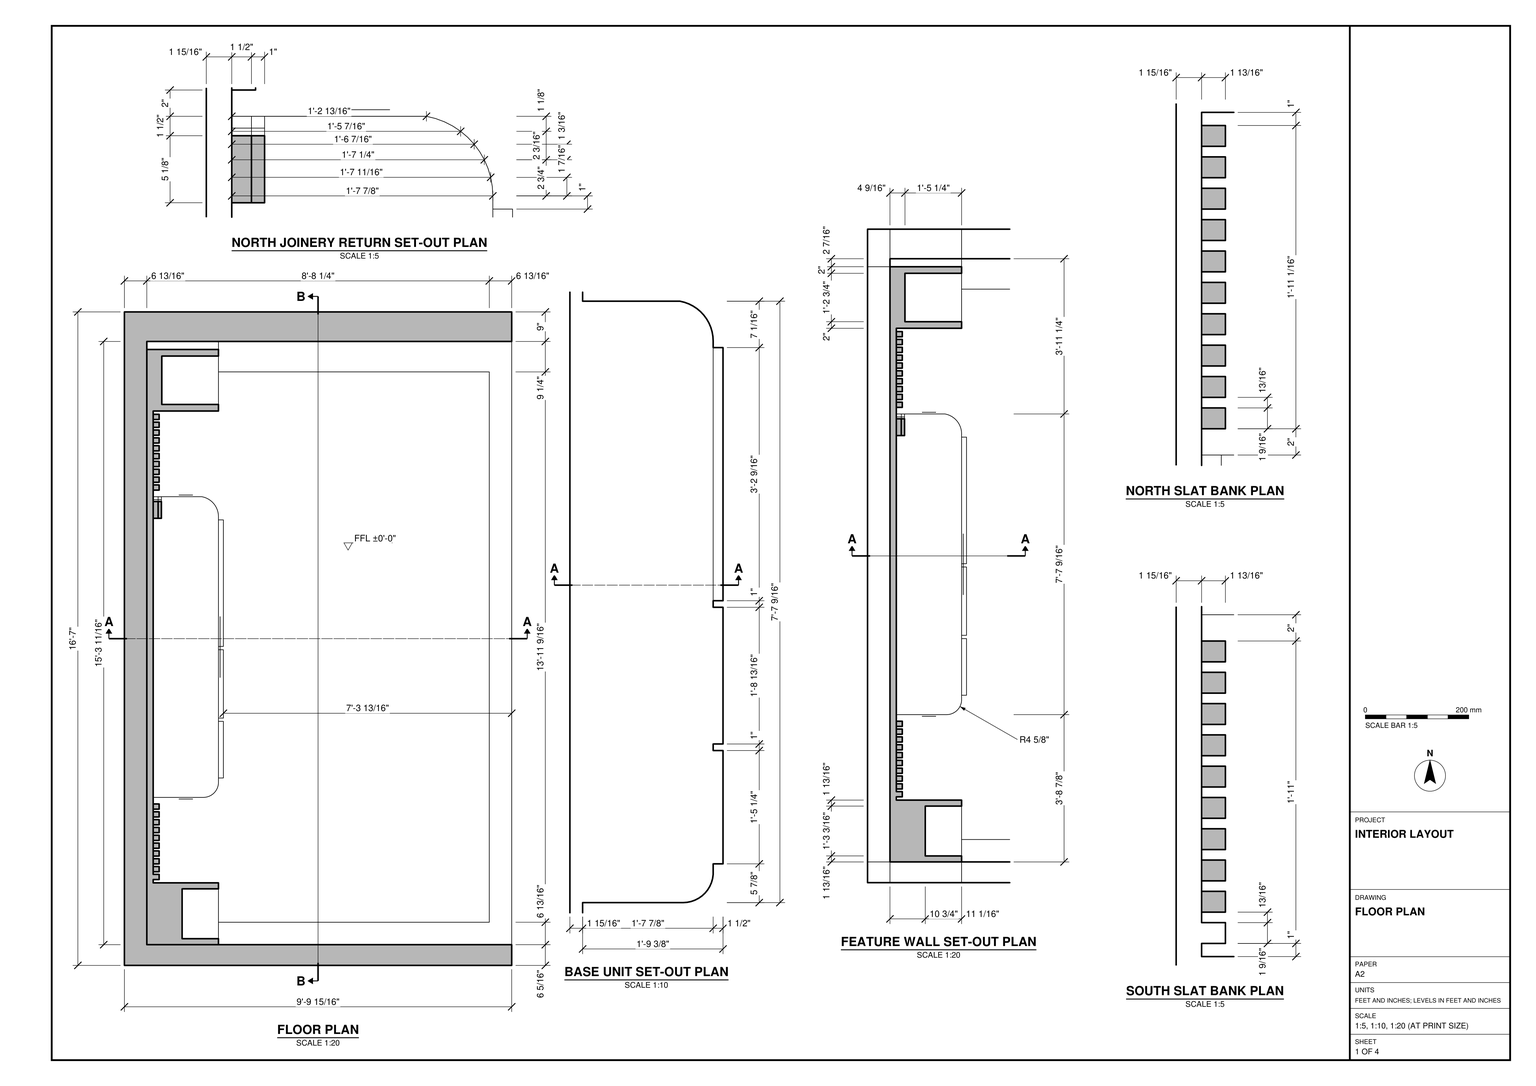
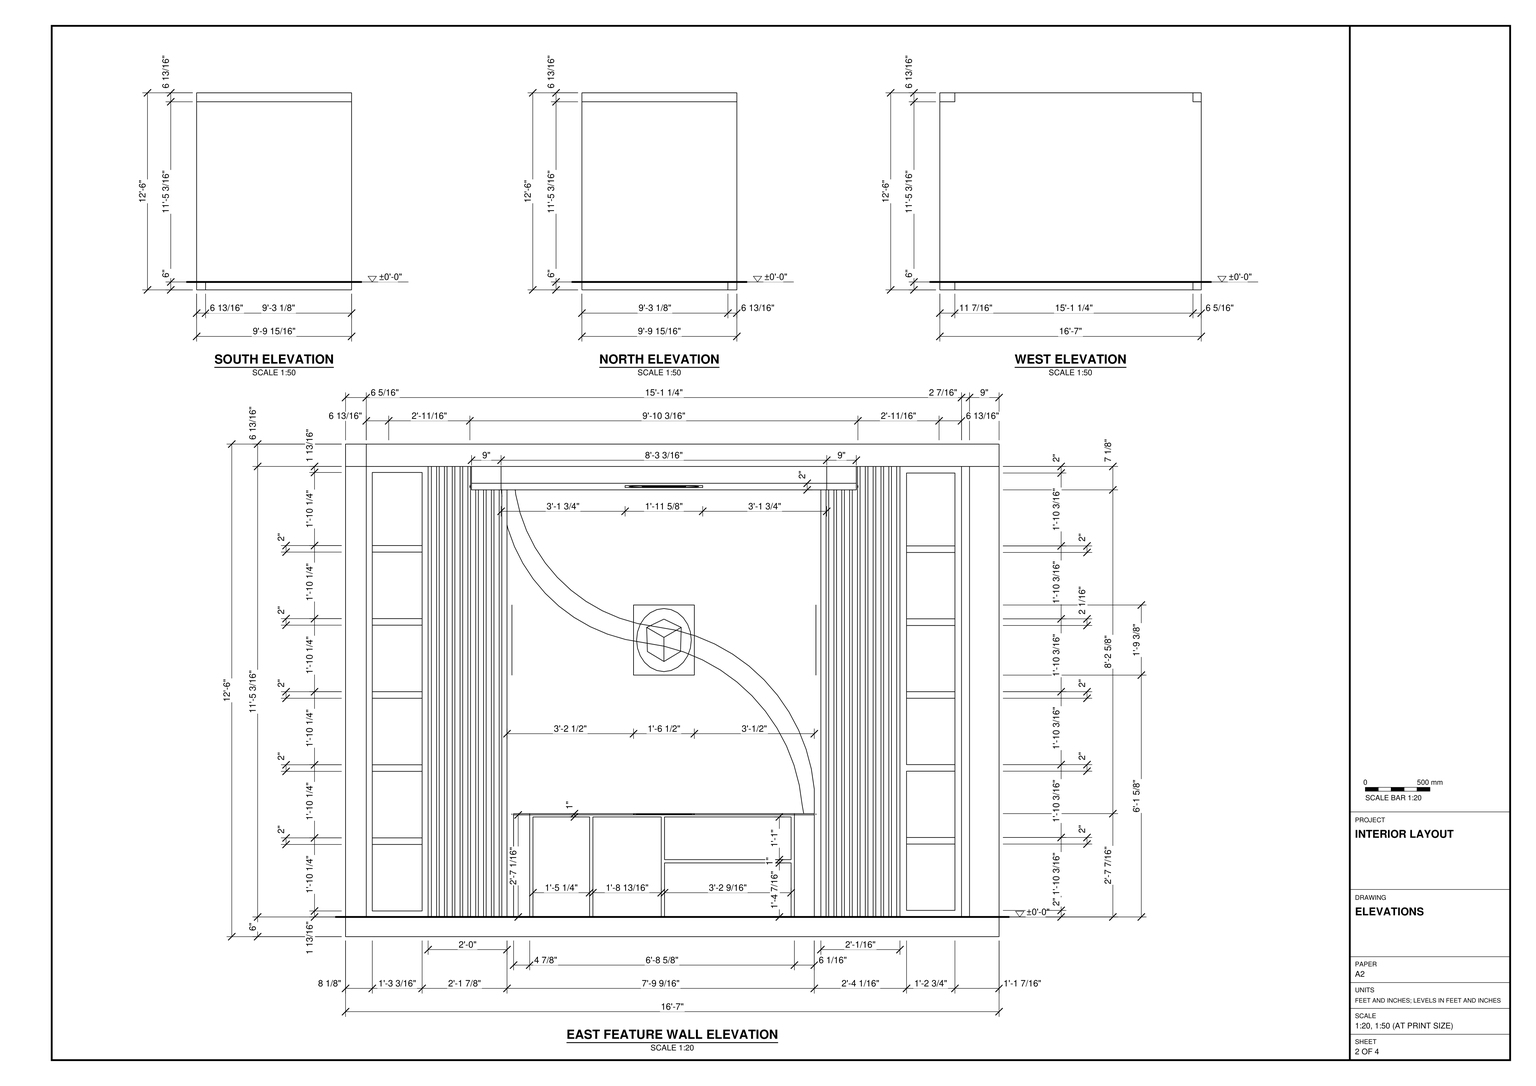
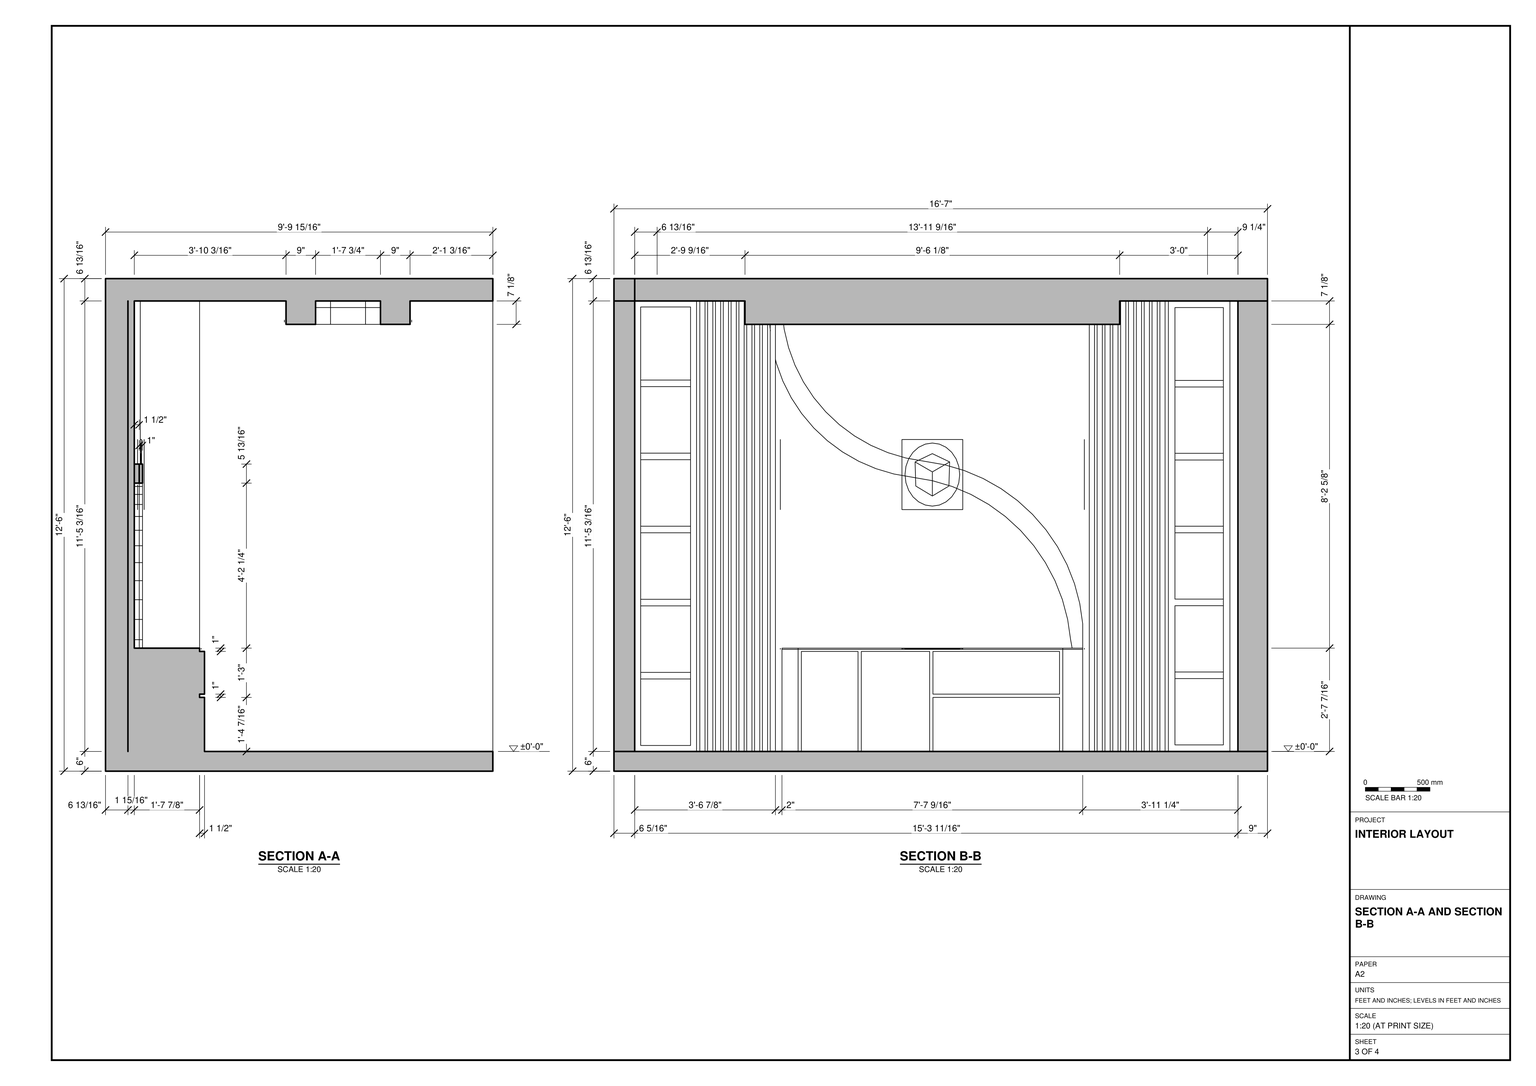
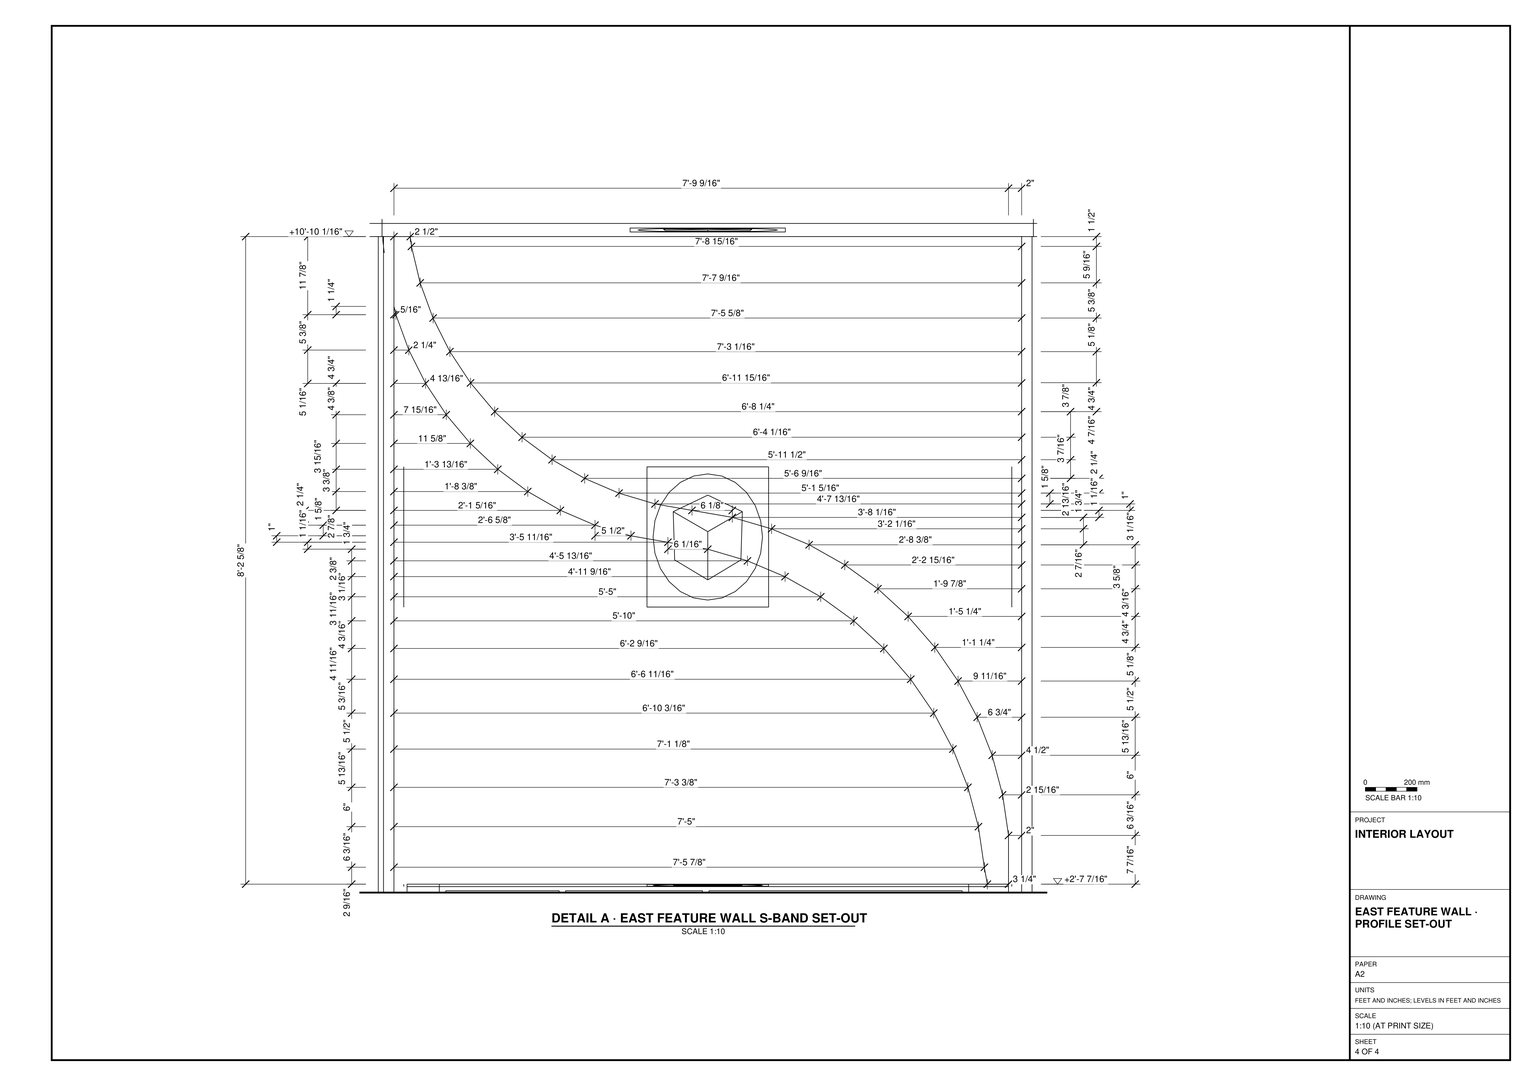
Build the room and its fitted joinery in SketchUp from task_files/diagram_01.pdf. Work in feet and inches. Set the finished floor at ±0'-0". The room shell measures 9'-9 15/16" east to west, 16'-7" north to south and 12'-6" high overall, including the floor and ceiling slabs.

Model the long west wall and the north and south end walls at their drawn thicknesses, leaving the east side open as shown in plan. Use the two sections to set the slab thicknesses and the position, depth and length of the ceiling projections. Keep the floor area in front of the joinery clear.

Build the east-facing feature wall using the elevation for the shelf heights and cabinet divisions, and the enlarged plans for the profiles. At each end, form a tall bank of open shelves with its own return depth. Place the closely spaced vertical slats between the shelves and the central panel. Run the curved band across the panel from the upper left to the lower right as seen in elevation, with the small wall-mounted feature near its centre. Below it, model the low base cabinet with its rounded front corners in plan and its divided front as drawn. Decor and loose items may be represented by any suitable library component.

Keep the walls, slabs and each joinery or furniture piece in separate groups or components, and use components for repeated parts such as matching slats. Save one SketchUp model as output_files/feature_wall_with_flanking_shelves_and_base_cabinetry.skp.

# SketchUp Ruby script. Lengths in inches.
U = 1.inch
M = Sketchup.active_model
def pt(a) = Geom::Point3d.new(a.map { |v| v * U })
def face(e, loops, mat)
  f = e.add_face(loops[0].map { |a| pt(a) })
  loops[1..].each { |l| e.add_face(l.map { |a| pt(a) }).erase! }
  f.material = f.back_material = mat if mat
  f
end
# faces: each face lists its corners as indices into pts; further lists are holes
def faces(e, pts, list, mat = nil) = list.each { |f| face(e, (f[0].is_a?(Array) ? f : [f]).map { |l| l.map { |i| pts[i] } }, mat) }
# xy, xz, yz: faces in a plane at the given z, y or x. An outline is a flat list of corners, or four numbers for a rectangle; further outlines are holes
def ring(l) = l.size == 4 ? [[l[0], l[1]], [l[2], l[1]], [l[2], l[3]], [l[0], l[3]]] : l.each_slice(2).to_a
def flat(e, list, mat, &to3) = list.each { |f| face(e, (f[0].is_a?(Array) ? f : [f]).map { |l| ring(l).map { |u, v| to3.(u, v) } }, mat) }
def xy(e, z, list, mat = nil) = flat(e, list, mat) { |x, y| [x, y, z] }
def xz(e, y, list, mat = nil) = flat(e, list, mat) { |x, z| [x, y, z] }
def yz(e, x, list, mat = nil) = flat(e, list, mat) { |y, z| [x, y, z] }
def lines(e, pts, list) = list.each { |a, b| e.add_line(pt(pts[a]), pt(pts[b])) }
# prism: a flat outline (further loops are holes) pulled along v
def prism(e, loops, v, mat = nil)
  f = face(e, loops, mat); d = Geom::Vector3d.new(v.map { |x| x * U })
  f.pushpull(f.normal.samedirection?(d) ? d.length : -d.length)
end
def box(e, o, s, mat = nil) = prism(e, [[o, [o[0] + s[0], o[1], o[2]], [o[0] + s[0], o[1] + s[1], o[2]], [o[0], o[1] + s[1], o[2]]]], [0, 0, s[2]], mat)
def at(x, y, z, deg = 0) = Geom::Transformation.translation(pt([x, y, z])) * Geom::Transformation.rotation(ORIGIN, Z_AXIS, deg.degrees)
def axes(o, x, y, z) = Geom::Transformation.new([*x, 0, *y, 0, *z, 0, *pt(o).to_a, 1])
def part(name) = M.definitions.add(name)
# library, detail: a bought-in or finely detailed component or shape, given as its bounding box
def library(name, o, s) = part(name).tap { |d| box(d.entities, o, s) }
def detail(e, o, s) = box(e.add_group.entities, o, s)
def put(e, d, t, mat = nil) = e.add_instance(d, t).tap { |i| i.material = mat if mat }
def group(e, t, mat = nil) = e.add_group.tap { |g| g.transformation = t; g.material = mat if mat }.entities
root = M.entities
M.materials.add("Marble Black 01 150cm").color = [30, 30, 30]
M.materials.add("Tiles Simple J01 100cm").color = [187, 218, 215]
M.materials.add("Wood Maple 33-40 200cm").color = [215, 177, 122]
M.materials.add("[Color D01]").color = [255, 242, 204]
M.materials.add("[Color F01]").color = [229, 255, 204]
M.materials.add("[Color M04]").color = [142, 142, 142]
c1 = library("Spot Light",[-5.1,-5.1,-11.05],[10.2,10.2,11.05])
c2 = library("Spot Light\#1",[-5.1,-5.1,-11.05],[10.2,10.2,11.05])
c3 = library("Group\#2",[0,0,0],[3,94.07,105.72])
c4 = library("Group\#3",[-0.5,-0.5,0],[20.875,92.57,0.375])
c5 = library("Group\#5",[-0.5,-0.5,0],[38.76,118.17,7.125])
c6 = library("Group\#6",[-0.5,-0.5,0],[20.76,100.17,2])
xy(root,0,[[0,0,0,187.5625,6.83,187.5625,6.83,199,117.9375,199,117.9375,0],[0,187.5625,6.83,199]])
xy(root,6,[[0,0,6.83,6.3125],[6.83,0,28.64,6.3125],[8.77,28.52,10.58,30.11],[8.77,30.9,10.58,32.49],[8.77,33.29,10.58,34.87],
  [8.77,35.67,10.58,37.25],[8.77,38.05,10.58,39.64],[8.77,40.43,10.58,42.02],[8.77,42.81,10.58,44.4],[8.77,45.2,10.58,46.78],
  [8.77,47.58,10.58,49.16],[8.77,144.73,10.58,146.32],[8.77,147.12,10.58,148.71],[8.77,149.51,10.58,151.1],[8.77,151.9,10.58,153.49],
  [8.77,154.29,10.58,155.875],[8.77,156.68,10.58,158.26],[8.77,159.07,10.58,160.65],[8.77,161.46,10.58,163.04],[8.77,163.85,10.58,165.43],
  [8.77,166.23,10.58,167.82],[0,187.5625,6.83,199],[6.83,187.5625,28.64,199]])
xy(root,6,[[28.64,0,117.9375,0,117.9375,199,28.64,199,28.64,180.73,111.11,180.73,111.11,13.14,28.64,13.14],[28.64,13.14,111.11,13.14,111.11,180.73,28.64,180.73,28.64,168.82,8.77,168.82,8.77,167.82,10.58,167.82,10.58,166.23,8.77,166.23,8.77,165.43,10.58,165.43,10.58,163.85,8.77,163.85,8.77,163.04,10.58,163.04,10.58,161.46,8.77,161.46,8.77,160.65,10.58,160.65,10.58,159.07,8.77,159.07,8.77,158.26,10.58,158.26,10.58,156.68,8.77,156.68,8.77,155.875,10.58,155.875,10.58,154.29,8.77,154.29,8.77,153.49,10.58,153.49,10.58,151.9,8.77,151.9,8.77,151.1,10.58,151.1,10.58,149.51,8.77,149.51,8.77,148.71,10.58,148.71,10.58,147.12,8.77,147.12,8.77,146.32,10.58,146.32,10.58,144.73,8.77,144.73,8.77,142.73,23.59,142.73,24.28,142.57,24.95,142.32,25.58,141.99,26.18,141.6,26.72,141.14,27.21,140.62,27.64,140.04,27.99,139.43,28.27,138.77,28.48,138.09,28.6,137.38,28.64,136.67,28.64,135.67,30.14,135.67,30.14,97.13,28.64,97.13,28.64,96.13,30.14,96.13,30.14,75.32,28.64,75.32,28.64,74.32,30.14,74.32,30.14,57.07,28.64,57.07,28.64,55.44,28.55,54.82,28.38,54.22,28.13,53.64,27.81,53.11,27.41,52.62,26.95,52.19,26.4375,51.83,25.88,51.54,25.29,51.33,24.68,51.21,24.05,51.16,8.77,51.16,8.77,49.16,10.58,49.16,10.58,47.58,8.77,47.58,8.77,46.78,10.58,46.78,10.58,45.2,8.77,45.2,8.77,44.4,10.58,44.4,10.58,42.81,8.77,42.81,8.77,42.02,10.58,42.02,10.58,40.43,8.77,40.43,8.77,39.64,10.58,39.64,10.58,38.05,8.77,38.05,8.77,37.25,10.58,37.25,10.58,35.67,8.77,35.67,8.77,34.87,10.58,34.87,10.58,33.29,8.77,33.29,8.77,32.49,10.58,32.49,10.58,30.9,8.77,30.9,8.77,30.11,10.58,30.11,10.58,28.52,8.77,28.52,8.77,27.73,10.58,27.73,10.58,26.14,8.77,26.14,8.77,25.14,28.64,25.14]],"Tiles Simple J01 100cm")
xy(root,7.83,[[17.58,8.14,28.64,13.14],[17.58,13.14,28.64,23.32]],"Marble Black 01 150cm")
xy(root,8,[[11.39,170.82,28.64,180.73],[11.39,180.73,28.64,185.5625]],"Marble Black 01 150cm")
xy(root,22.46,[[28.64,97.13,30.14,135.67]],"Wood Maple 33-40 200cm")
xy(root,23.46,[[28.64,97.13,30.14,135.67]])
xy(root,28.08,[[17.58,8.14,28.64,23.32]],"Marble Black 01 150cm")
xy(root,28.2,[[11.39,170.82,28.64,185.5625]],"Marble Black 01 150cm")
xy(root,30.08,[[17.58,8.14,28.64,23.32]],"Marble Black 01 150cm")
xy(root,30.2,[[11.39,170.82,28.64,185.5625]],"Marble Black 01 150cm")
xy(root,36.46,[[28.64,97.13,30.14,135.67]])
xy(root,36.46,[[28.64,57.07,30.14,74.32],[28.64,75.32,30.14,96.13]],"Wood Maple 33-40 200cm")
xy(root,37.46,[[8.77,51.16,24.05,51.16,24.68,51.21,25.29,51.33,25.88,51.54,26.4375,51.83,26.95,52.19,27.41,52.62,27.81,53.11,28.13,53.64,28.38,54.22,28.55,54.82,28.64,55.44,28.64,136.67,28.6,137.38,28.48,138.09,28.27,138.77,27.99,139.43,27.64,140.04,27.21,140.62,26.72,141.14,26.18,141.6,25.58,141.99,24.95,142.32,24.28,142.57,23.59,142.73,8.77,142.73]],"Wood Maple 33-40 200cm")
xy(root,50.34,[[17.58,8.14,28.64,23.32]],"Marble Black 01 150cm")
xy(root,52.34,[[17.58,8.14,28.64,23.32]],"Marble Black 01 150cm")
xy(root,52.4,[[11.39,170.82,28.64,185.5625]],"Marble Black 01 150cm")
xy(root,72.59,[[17.58,8.14,28.64,23.32]],"Marble Black 01 150cm")
xy(root,72.6,[[11.39,170.82,28.64,185.5625]],"Marble Black 01 150cm")
xy(root,74.59,[[17.58,8.14,28.64,23.32],[11.39,170.82,28.64,185.5625]],"Marble Black 01 150cm")
xy(root,94.75,[[11.39,170.82,28.64,185.5625]],"Marble Black 01 150cm")
xy(root,94.85,[[17.58,8.14,28.64,23.32]],"Marble Black 01 150cm")
xy(root,96.79,[[11.39,170.82,28.64,185.5625]],"Marble Black 01 150cm")
xy(root,96.85,[[17.58,8.14,28.64,23.32]],"Marble Black 01 150cm")
xy(root,116.99,[[11.39,170.82,28.64,185.5625]],"Marble Black 01 150cm")
xy(root,117.11,[[17.58,8.14,28.64,23.32]],"Marble Black 01 150cm")
xy(root,118.99,[[11.39,170.82,28.64,185.5625]])
xy(root,119.11,[[17.58,8.14,28.64,23.32]],"Marble Black 01 150cm")
xy(root,141.1875,[[11.39,170.82,28.64,180.73],[11.39,180.73,28.64,185.5625]],"Marble Black 01 150cm")
xy(root,141.36,[[17.58,8.14,28.64,13.14],[17.58,13.14,28.64,23.32]],"Marble Black 01 150cm")
xy(root,143.1875,[[0,0,6.83,6.3125],[6.83,0,28.64,6.3125],[8.77,28.52,10.58,30.11],[8.77,30.9,10.58,32.49],[8.77,33.29,10.58,34.87],
  [8.77,35.67,10.58,37.25],[8.77,38.05,10.58,39.64],[8.77,40.43,10.58,42.02],[8.77,42.81,10.58,44.4],[8.77,45.2,10.58,46.78],
  [8.77,47.58,10.58,49.16],[8.77,144.73,10.58,146.32],[8.77,147.12,10.58,148.71],[8.77,149.51,10.58,151.1],[8.77,151.9,10.58,153.49],
  [8.77,154.29,10.58,155.875],[8.77,156.68,10.58,158.26],[8.77,159.07,10.58,160.65],[8.77,161.46,10.58,163.04],[8.77,163.85,10.58,165.43],
  [8.77,166.23,10.58,167.82],[0,187.5625,6.83,199],[6.83,187.5625,28.64,199]])
xy(root,143.1875,[[28.64,0,117.9375,13.14],[28.64,180.73,117.9375,199]],"[Color D01]")
xy(root,150,[[0,0,117.9375,199]])
xz(root,0,[[0,0,6.83,6],[6.83,0,117.9375,6],[0,143.1875,117.9375,150]])
xz(root,6.3125,[[6.83,6,28.64,143.1875],[0,143.1875,117.9375,150]])
xz(root,8.14,[[17.58,7.83,28.64,28.08],[17.58,30.08,28.64,50.34],[17.58,52.34,28.64,72.59],[17.58,74.59,28.64,94.85],[17.58,96.85,28.64,117.11],
  [17.58,119.11,28.64,141.36]],"Marble Black 01 150cm")
xz(root,23.32,[[17.58,28.08,28.64,30.08],[17.58,50.34,28.64,52.34],[17.58,72.59,28.64,74.59],[17.58,74.59,28.64,94.85],[17.58,94.85,28.64,96.85],
  [17.58,117.11,28.64,119.11]])
xz(root,23.32,[[17.58,7.83,28.64,28.08],[17.58,30.08,28.64,50.34],[17.58,52.34,28.64,72.59],[17.58,96.85,28.64,117.11],[17.58,119.11,28.64,141.36]],"Marble Black 01 150cm")
xz(root,25.14,[[8.77,6,28.64,143.1875]],"Marble Black 01 150cm")
xz(root,26.14,[[8.77,6,10.58,143.1875]],"Wood Maple 33-40 200cm")
xz(root,27.73,[[8.77,6,10.58,143.1875]],"Wood Maple 33-40 200cm")
xz(root,28.52,[[8.77,6,10.58,143.1875]],"Wood Maple 33-40 200cm")
xz(root,30.11,[[8.77,6,10.58,143.1875]],"Wood Maple 33-40 200cm")
xz(root,30.9,[[8.77,6,10.58,143.1875]],"Wood Maple 33-40 200cm")
xz(root,32.49,[[8.77,6,10.58,143.1875]],"Wood Maple 33-40 200cm")
xz(root,33.29,[[8.77,6,10.58,143.1875]],"Wood Maple 33-40 200cm")
xz(root,34.87,[[8.77,6,10.58,143.1875]],"Wood Maple 33-40 200cm")
xz(root,35.67,[[8.77,6,10.58,143.1875]],"Wood Maple 33-40 200cm")
xz(root,37.25,[[8.77,6,10.58,143.1875]],"Wood Maple 33-40 200cm")
xz(root,38.05,[[8.77,6,10.58,143.1875]],"Wood Maple 33-40 200cm")
xz(root,39.64,[[8.77,6,10.58,143.1875]],"Wood Maple 33-40 200cm")
xz(root,40.43,[[8.77,6,10.58,143.1875]],"Wood Maple 33-40 200cm")
xz(root,42.02,[[8.77,6,10.58,143.1875]],"Wood Maple 33-40 200cm")
xz(root,42.81,[[8.77,6,10.58,143.1875]],"Wood Maple 33-40 200cm")
xz(root,44.4,[[8.77,6,10.58,143.1875]],"Wood Maple 33-40 200cm")
xz(root,45.2,[[8.77,6,10.58,143.1875]],"Wood Maple 33-40 200cm")
xz(root,46.78,[[8.77,6,10.58,143.1875]],"Wood Maple 33-40 200cm")
xz(root,47.58,[[8.77,6,10.58,143.1875]],"Wood Maple 33-40 200cm")
xz(root,49.16,[[8.77,6,10.58,143.1875]],"Wood Maple 33-40 200cm")
xz(root,51.16,[[8.77,6,24.05,37.09]],"Wood Maple 33-40 200cm")
xz(root,57.07,[[28.64,6,30.14,36.46]],"Wood Maple 33-40 200cm")
xz(root,74.32,[[28.64,6,30.14,36.46]])
xz(root,75.32,[[28.64,6,30.14,36.46]],"Wood Maple 33-40 200cm")
xz(root,96.13,[[28.64,6,30.14,36.46]],"Wood Maple 33-40 200cm")
xz(root,97.13,[[28.64,6,30.14,22.46],[28.64,23.46,30.14,36.46]])
xz(root,135.67,[[28.64,6,30.14,22.46],[28.64,23.46,30.14,36.46]],"Wood Maple 33-40 200cm")
xz(root,142.73,[[8.77,6,23.59,37.09]],"Wood Maple 33-40 200cm")
xz(root,144.73,[[8.77,6,10.58,143.1875]],"Wood Maple 33-40 200cm")
xz(root,146.32,[[8.77,6,10.58,143.1875]],"Wood Maple 33-40 200cm")
xz(root,147.12,[[8.77,6,10.58,143.1875]],"Wood Maple 33-40 200cm")
xz(root,148.71,[[8.77,6,10.58,143.1875]],"Wood Maple 33-40 200cm")
xz(root,149.51,[[8.77,6,10.58,143.1875]],"Wood Maple 33-40 200cm")
xz(root,151.1,[[8.77,6,10.58,143.1875]],"Wood Maple 33-40 200cm")
xz(root,151.9,[[8.77,6,10.58,143.1875]],"Wood Maple 33-40 200cm")
xz(root,153.49,[[8.77,6,10.58,143.1875]],"Wood Maple 33-40 200cm")
xz(root,154.29,[[8.77,6,10.58,143.1875]],"Wood Maple 33-40 200cm")
xz(root,155.875,[[8.77,6,10.58,143.1875]],"Wood Maple 33-40 200cm")
xz(root,156.68,[[8.77,6,10.58,143.1875]],"Wood Maple 33-40 200cm")
xz(root,158.26,[[8.77,6,10.58,143.1875]],"Wood Maple 33-40 200cm")
xz(root,159.07,[[8.77,6,10.58,143.1875]],"Wood Maple 33-40 200cm")
xz(root,160.65,[[8.77,6,10.58,143.1875]],"Wood Maple 33-40 200cm")
xz(root,161.46,[[8.77,6,10.58,143.1875]],"Wood Maple 33-40 200cm")
xz(root,163.04,[[8.77,6,10.58,143.1875]],"Wood Maple 33-40 200cm")
xz(root,163.85,[[8.77,6,10.58,143.1875]],"Wood Maple 33-40 200cm")
xz(root,165.43,[[8.77,6,10.58,143.1875]],"Wood Maple 33-40 200cm")
xz(root,166.23,[[8.77,6,10.58,143.1875]],"Wood Maple 33-40 200cm")
xz(root,167.82,[[8.77,6,10.58,143.1875]],"Wood Maple 33-40 200cm")
xz(root,168.82,[[8.77,6,28.64,143.1875]],"Marble Black 01 150cm")
xz(root,170.82,[[11.39,8,28.64,28.2],[11.39,30.2,11.39,50.4,28.64,50.39,28.64,30.2],[11.39,52.4,28.64,72.6],[11.39,74.59,28.64,94.75],[11.39,96.79,28.64,116.99],
  [11.39,118.99,28.64,141.1875]],"Marble Black 01 150cm")
xz(root,185.5625,[[11.39,28.2,28.64,30.2],[28.64,50.39,11.39,50.4,11.39,52.4,28.64,52.4],[11.39,72.6,28.64,74.59],[11.39,94.75,28.64,96.79],[11.39,116.99,28.64,118.99]])
xz(root,185.5625,[[11.39,8,28.64,28.2],[11.39,30.2,28.64,30.2,28.64,50.39,11.39,50.4],[11.39,52.4,28.64,72.6],[11.39,74.59,28.64,94.75],[11.39,96.79,28.64,116.99],
  [11.39,118.99,28.64,141.1875]],"Marble Black 01 150cm")
xz(root,187.5625,[[0,0,6.83,6],[6.83,6,28.64,143.1875]])
xz(root,199,[[0,0,6.83,6],[6.83,0,117.9375,6],[0,143.1875,117.9375,150]])
yz(root,0,[[0,0,6.3125,6],[187.5625,0,199,6],[0,143.1875,6.3125,150],[187.5625,143.1875,199,150]])
yz(root,6.83,[[6.3125,6,13.14,143.1875],[180.73,6,187.5625,143.1875]])
yz(root,8.77,[[25.14,6,26.14,143.1875],[27.73,6,28.52,143.1875],[28.52,6,30.11,143.1875],[30.11,6,30.9,143.1875],[30.9,6,32.49,143.1875],
  [32.49,6,33.29,143.1875],[33.29,6,34.87,143.1875],[34.87,6,35.67,143.1875],[35.67,6,37.25,143.1875],[37.25,6,38.05,143.1875],
  [38.05,6,39.64,143.1875],[39.64,6,40.43,143.1875],[42.02,6,42.81,143.1875],[42.81,6,44.4,143.1875],[44.4,6,45.2,143.1875],
  [45.2,6,46.78,143.1875],[46.78,6,47.58,143.1875],[47.58,6,49.16,6,49.16,125.4375,48.15,129.72,47.58,134.54],[144.73,6,146.32,143.1875],[146.32,6,147.12,143.1875],
  [147.12,6,148.71,143.1875],[148.71,6,149.51,143.1875],[149.51,6,151.1,143.1875],[151.1,6,151.9,143.1875],[151.9,6,153.49,143.1875],
  [153.49,6,154.29,143.1875],[154.29,6,155.875,143.1875],[155.875,6,156.68,143.1875],[156.68,6,158.26,143.1875],[158.26,6,159.07,143.1875],
  [159.07,6,160.65,143.1875],[160.65,6,161.46,143.1875],[161.46,6,163.04,143.1875],[163.04,6,163.85,143.1875],[163.85,6,165.43,143.1875],
  [165.43,6,166.23,143.1875],[166.23,6,167.82,143.1875],[167.82,6,168.82,143.1875],[49.16,125.4375,49.16,143.1875,47.58,143.1875,47.58,134.54,48.15,129.72]])
yz(root,8.77,[[40.43,6,42.02,143.1875]],"Wood Maple 33-40 200cm")
yz(root,8.77,[[49.16,6,51.16,6,51.16,37.46,139.51,37.46,139.05,40.04,138.15,46.2,136.55,52.22,134.28,58.02,131.37,63.52,127.84,68.66,123.76,73.36,119.17,77.5625,114.13,81.22,108.71,84.28,102.97,86.7,97,88.45,90.86,89.52,85.24,90.5,79.76,92.13,74.51,94.38,69.5625,97.23,64.98,100.64,60.82,104.55,57.14,108.92,53.99,113.69,51.43,118.8,49.47,124.16,49.16,125.4375],[142.73,6,144.73,6,144.73,143.1875,51.16,143.1875,51.16,140.25,51.83,134.58,53.15,129.02,55.11,123.65,57.68,118.55,60.82,113.78,64.5,109.41,68.66,105.5,73.25,102.09,78.2,99.24,83.45,96.99,88.92,95.36,94.55,94.375,100.68,93.3125,106.66,91.56,112.39,89.13,117.82,86.08,122.86,82.42,127.45,78.21,131.53,73.51,135.05,68.38,137.97,62.875,140.24,57.08,141.83,51.0625,142.73,44.9]],"[Color F01]")
yz(root,10.58,[[26.14,6,27.73,143.1875],[28.52,6,30.11,143.1875],[30.9,6,32.49,143.1875],[33.29,6,34.87,143.1875],[35.67,6,37.25,143.1875],
  [38.05,6,39.64,143.1875],[40.43,6,42.02,143.1875],[42.81,6,44.4,143.1875],[45.2,6,46.78,143.1875],[47.58,6,49.16,143.1875],
  [144.73,6,146.32,143.1875],[147.12,6,148.71,143.1875],[149.51,6,151.1,143.1875],[151.9,6,153.49,143.1875],[154.29,6,155.875,143.1875],
  [156.68,6,158.26,143.1875],[159.07,6,160.65,143.1875],[161.46,6,163.04,143.1875],[163.85,6,165.43,143.1875],[166.23,6,167.82,143.1875]],"Wood Maple 33-40 200cm")
yz(root,11.39,[[170.82,8,185.5625,28.2],[170.82,30.2,185.5625,50.4],[170.82,52.4,185.5625,72.6],[170.82,74.59,185.5625,94.75],[170.82,96.79,185.5625,116.99],
  [170.82,118.99,185.5625,141.1875]],"Marble Black 01 150cm")
yz(root,17.58,[[8.14,7.83,23.32,28.08],[8.14,30.08,23.32,50.34],[8.14,52.34,23.32,72.59],[8.14,74.59,23.32,94.85],[8.14,96.85,23.32,117.11],
  [8.14,119.11,23.32,141.36]],"Marble Black 01 150cm")
yz(root,28.64,[[[6.3125,6,25.14,143.1875],[8.14,7.83,8.14,141.36,23.32,141.36,23.32,119.11,8.14,119.11,8.14,117.11,23.32,117.11,23.32,96.85,8.14,96.85,8.14,94.85,23.32,94.85,23.32,74.59,8.14,74.59,8.14,72.59,23.32,72.59,23.32,52.34,8.14,52.34,8.14,50.34,23.32,50.34,23.32,30.08,8.14,30.08,8.14,28.08,23.32,28.08,23.32,7.83]],[[168.82,6,187.5625,143.1875],[170.82,52.4,170.82,141.1875,185.5625,141.1875,185.5625,118.99,170.82,118.99,170.82,116.99,185.5625,116.99,185.5625,96.79,170.82,96.79,170.82,94.75,185.5625,94.75,185.5625,74.59,170.82,74.59,170.82,72.6,185.5625,72.6,185.5625,52.4],[170.82,8,170.82,50.39,185.5625,50.39,185.5625,30.2,170.82,30.2,170.82,28.2,185.5625,28.2,185.5625,8]]],"Marble Black 01 150cm")
yz(root,28.64,[[55.44,6,56.07,37.09],[[56.07,6,57.07,6,57.07,36.46,74.32,36.46,74.32,6,75.32,6,75.32,36.46,96.13,36.46,96.13,6,97.13,6,97.13,22.46,135.67,22.46,135.67,6,136.67,6,136.67,37.09,56.07,37.09],[97.13,23.46,135.67,36.46]]],"Wood Maple 33-40 200cm")
yz(root,30.14,[[57.07,6,74.32,36.46],[75.32,6,96.13,36.46],[97.13,6,135.67,22.46],[97.13,23.46,135.67,36.46]],"Wood Maple 33-40 200cm")
yz(root,117.9375,[[0,143.1875,199,150]])
yz(root,117.9375,[[0,0,199,6]],"Tiles Simple J01 100cm")
p = [[24.68,51.21,6],[24.68,51.21,37.09],[24.05,51.16,37.09],[24.05,51.16,6],[25.29,51.33,6],[25.29,51.33,37.09],
  [25.88,51.54,6],[25.88,51.54,37.09],[26.4375,51.83,6],[26.4375,51.83,37.09],[26.95,52.19,6],[26.95,52.19,37.09],
  [27.41,52.62,6],[27.41,52.62,37.09],[27.81,53.11,6],[27.81,53.11,37.09],[28.13,53.64,6],[28.13,53.64,37.09],
  [28.38,54.22,6],[28.38,54.22,37.09],[28.55,54.82,6],[28.55,54.82,37.09],[28.64,55.44,6],[28.64,55.44,37.09],
  [28.6,137.38,6],[28.6,137.38,37.09],[28.64,136.67,37.09],[28.64,136.67,6],[28.48,138.09,6],[28.48,138.09,37.09],
  [28.27,138.77,6],[28.27,138.77,37.09],[27.99,139.43,6],[27.99,139.43,37.09],[27.64,140.04,6],[27.64,140.04,37.09],
  [27.21,140.62,6],[27.21,140.62,37.09],[26.72,141.14,6],[26.72,141.14,37.09],[26.18,141.6,6],[26.18,141.6,37.09],
  [25.58,141.99,6],[25.58,141.99,37.09],[24.95,142.32,6],[24.95,142.32,37.09],[24.28,142.57,6],[24.28,142.57,37.09],
  [23.59,142.73,6],[23.59,142.73,37.09],[28.64,170.82,50.39],[11.39,170.82,50.4],[11.39,185.5625,50.4],[28.64,185.5625,50.39],
  [8.77,47.48,135.39],[8.77,47.58,134.54],[8.77,47.48,138.33]]
faces(root,p,[[0,1,2,3],[4,5,1,0],[6,7,5,4],[8,9,7,6],[10,11,9,8],[12,13,11,10],[14,15,13,12],[16,17,15,14],
  [18,19,17,16],[20,21,19,18],[22,23,21,20],[24,25,26,27],[28,29,25,24],[30,31,29,28],[32,33,31,30],[34,35,33,32],
  [36,37,35,34],[38,39,37,36],[40,41,39,38],[42,43,41,40],[44,45,43,42],[46,47,45,44],[48,49,47,46]],"Wood Maple 33-40 200cm")
faces(root,p,[[50,51,52,53]],"Marble Black 01 150cm")
lines(root,p,[[54,55],[54,56]])
put(root,c1,at(27.43,15.75,140.35))
put(root,c1,at(25.35,15.17,117.11))
put(root,c1,at(25.35,15.17,92.86))
put(root,c1,at(25.35,15.17,72.04))
put(root,c1,at(25.35,15.17,49.23))
put(root,c1,at(25.35,15.17,26.86))
put(root,c2,at(26.71,177.97,140.18))
put(root,c2,at(26.71,177.97,116.18))
put(root,c2,at(26.71,177.97,93.12))
put(root,c2,at(26.71,177.97,71.74))
put(root,c2,at(26.71,177.97,48.12))
put(root,c2,at(26.71,177.97,27.18))
g1 = group(root,at(0,6.3125,0),"Wood Maple 33-40 200cm")
xy(g1,6,[[0,-6.3125,117.9375,0],[0,181.25,0,192.6875,117.9375,192.6875,117.9375,183.6875,6.83,183.6875,6.83,181.25]])
xy(g1,143.1875,[[0,-6.3125,117.9375,0],[0,181.25,6.83,181.25,6.83,183.6875,117.9375,183.6875,117.9375,192.6875,0,192.6875]])
xz(g1,-6.3125,[[0,6,117.9375,143.1875]],"[Color D01]")
xz(g1,0,[[6.83,6,117.9375,143.1875]],"[Color D01]")
xz(g1,183.6875,[[6.83,6,117.9375,143.1875]],"[Color D01]")
xz(g1,192.6875,[[0,6,117.9375,143.1875]],"[Color D01]")
yz(g1,0,[[0,0,0,6,-6.3125,6,-6.3125,143.1875,0,143.1875,0,150,181.25,150,181.25,143.1875,192.6875,143.1875,192.6875,6,181.25,6,181.25,0]])
yz(g1,6.83,[[0,6,6.83,143.1875],[6.83,6,174.42,143.1875],[174.42,6,183.6875,143.1875]])
yz(g1,117.9375,[[-6.3125,6,0,143.1875],[183.6875,6,192.6875,143.1875]],"[Color D01]")
put(root,c3,at(8.77,49.16,37.46))
put(root,c4,at(8.77,51.16,37.09))
g2 = group(root,at(8.77,13.14,143.1875))
xy(g2,0,[[19.875,0,19.875,12,0,12,0,13,1.8125,13,1.8125,14.59,0,14.59,0,15.38,1.8125,15.38,1.8125,16.97,0,16.97,0,17.76,1.8125,17.76,1.8125,19.35,0,19.35,0,20.15,1.8125,20.15,1.8125,21.73,0,21.73,0,22.53,1.8125,22.53,1.8125,24.11,0,24.11,0,24.91,1.8125,24.91,1.8125,26.49,0,26.49,0,27.29,1.8125,27.29,1.8125,28.875,0,28.875,0,29.67,1.8125,29.67,1.8125,31.26,0,31.26,0,32.06,1.8125,32.06,1.8125,33.64,0,33.64,0,34.4375,1.8125,34.4375,1.8125,36.02,0,36.02,0,131.59,1.8125,131.59,1.8125,133.18,0,133.18,0,133.98,1.8125,133.98,1.8125,135.57,0,135.57,0,136.37,1.8125,136.37,1.8125,137.96,0,137.96,0,138.76,1.8125,138.76,1.8125,140.34,0,140.34,0,141.15,1.8125,141.15,1.8125,142.73,0,142.73,0,143.54,1.8125,143.54,1.8125,145.12,0,145.12,0,145.93,1.8125,145.93,1.8125,147.51,0,147.51,0,148.32,1.8125,148.32,1.8125,149.9,0,149.9,0,150.7,1.8125,150.7,1.8125,152.29,0,152.29,0,153.09,1.8125,153.09,1.8125,154.68,0,154.68,0,155.68,19.875,155.68,19.875,167.59,20.98,167.59,20.98,0],[[20.98,0,109.17,167.59],[27.97,6.98,102.1875,160.61]],[[27.97,6.98,102.1875,160.61],[55.2,25.21,77.15,25.21,78.1,25.54,79.02,25.97,79.88,26.49,80.68,27.1,81.41,27.8,82.0625,28.57,82.63,29.41,83.1,30.3,83.47,31.24,83.74,32.21,83.9,33.21,83.96,34.21,83.96,133.38,83.9,134.39,83.74,135.38,83.47,136.36,83.1,137.29,82.63,138.1875,82.0625,139.02,81.41,139.79,80.68,140.49,79.88,141.1,79.02,141.625,78.1,142.05,77.15,142.38,55.2,142.38,54.02,142.3,52.87,142.07,51.75,141.69,50.7,141.17,49.72,140.52,48.83,139.74,48.06,138.86,47.4,137.88,46.88,136.82,46.5,135.71,46.27,134.55,46.2,133.38,46.2,34.21,46.27,33.04,46.5,31.88,46.88,30.77,47.4,29.71,48.06,28.73,48.83,27.85,49.72,27.07,50.7,26.42,51.75,25.9,52.87,25.52,54.02,25.29]]],"[Color D01]")
xy(g2,0,[[60.14,34.21,59.5,34.26,58.86,34.38,58.25,34.59,57.67,34.875,57.13,35.24,56.65,35.66,56.22,36.15,55.86,36.6875,55.57,37.27,55.37,37.88,55.24,38.51,55.2,39.16,55.2,128.83,55.24,129.42,55.35,130,55.54,130.57,55.81,131.1,56.14,131.6,56.53,132.05,56.98,132.4375,57.47,132.77,58.01,133.03,58.57,133.22,59.16,133.34,59.75,133.38,70.4,133.38,71,133.34,71.58,133.22,72.15,133.03,72.68,132.77,73.18,132.4375,73.625,132.05,74.02,131.6,74.35,131.1,74.61,130.57,74.8,130,74.92,129.42,74.96,128.83,74.96,38.32,74.92,37.79,74.82,37.26,74.65,36.75,74.41,36.27,74.11,35.82,73.75,35.42,73.35,35.0625,72.9,34.76,72.42,34.53,71.91,34.35,71.38,34.25,70.85,34.21]],"[Color M04]")
xz(g2,25.21,[[55.2,-5.125,77.15,0]],"[Color M04]")
xz(g2,142.38,[[55.2,-5.125,77.15,0]],"[Color M04]")
yz(g2,46.2,[[34.21,-5.125,133.38,0]],"[Color M04]")
yz(g2,83.96,[[34.21,-5.125,133.38,0]],"[Color M04]")
p = [[54.02,25.29,0],[54.02,25.29,-5.125],[55.2,25.21,-5.125],[55.2,25.21,0],[77.15,25.21,0],[77.15,25.21,-5.125],
  [78.1,25.54,-5.125],[78.1,25.54,0],[52.87,25.52,0],[52.87,25.52,-5.125],[51.75,25.9,0],[51.75,25.9,-5.125],
  [79.02,25.97,-5.125],[79.02,25.97,0],[50.7,26.42,0],[50.7,26.42,-5.125],[79.88,26.49,-5.125],[79.88,26.49,0],
  [49.72,27.07,0],[49.72,27.07,-5.125],[80.68,27.1,-5.125],[80.68,27.1,0],[48.83,27.85,0],[48.83,27.85,-5.125],
  [81.41,27.8,-5.125],[81.41,27.8,0],[48.06,28.73,0],[48.06,28.73,-5.125],[82.0625,28.57,-5.125],[82.0625,28.57,0],
  [82.63,29.41,-5.125],[82.63,29.41,0],[47.4,29.71,0],[47.4,29.71,-5.125],[83.1,30.3,-5.125],[83.1,30.3,0],
  [46.88,30.77,0],[46.88,30.77,-5.125],[83.47,31.24,-5.125],[83.47,31.24,0],[46.5,31.88,0],[46.5,31.88,-5.125],
  [83.74,32.21,-5.125],[83.74,32.21,0],[46.27,33.04,0],[46.27,33.04,-5.125],[83.9,33.21,-5.125],[83.9,33.21,0],
  [46.2,34.21,0],[46.2,34.21,-5.125],[83.96,34.21,-5.125],[83.96,34.21,0],[46.27,134.55,0],[46.27,134.55,-5.125],
  [46.2,133.38,-5.125],[46.2,133.38,0],[83.96,133.38,0],[83.96,133.38,-5.125],[83.9,134.39,-5.125],[83.9,134.39,0],
  [83.74,135.38,-5.125],[83.74,135.38,0],[46.5,135.71,0],[46.5,135.71,-5.125],[83.47,136.36,-5.125],[83.47,136.36,0],
  [46.88,136.82,0],[46.88,136.82,-5.125],[83.1,137.29,-5.125],[83.1,137.29,0],[47.4,137.88,0],[47.4,137.88,-5.125],
  [82.63,138.1875,-5.125],[82.63,138.1875,0],[48.06,138.86,0],[48.06,138.86,-5.125],[82.0625,139.02,-5.125],[82.0625,139.02,0],
  [48.83,139.74,0],[48.83,139.74,-5.125],[81.41,139.79,-5.125],[81.41,139.79,0],[49.72,140.52,0],[49.72,140.52,-5.125],
  [80.68,140.49,-5.125],[80.68,140.49,0],[50.7,141.17,0],[50.7,141.17,-5.125],[79.88,141.1,-5.125],[79.88,141.1,0],
  [79.02,141.625,-5.125],[79.02,141.625,0],[51.75,141.69,0],[51.75,141.69,-5.125],[78.1,142.05,-5.125],[78.1,142.05,0],
  [52.87,142.07,0],[52.87,142.07,-5.125],[54.02,142.3,0],[54.02,142.3,-5.125],[77.15,142.38,-5.125],[77.15,142.38,0],
  [55.2,142.38,0],[55.2,142.38,-5.125]]
faces(g2,p,[[0,1,2,3],[4,5,6,7],[8,9,1,0],[10,11,9,8],[7,6,12,13],[14,15,11,10],[13,12,16,17],[18,19,15,14],
  [17,16,20,21],[22,23,19,18],[21,20,24,25],[26,27,23,22],[25,24,28,29],[29,28,30,31],[32,33,27,26],[31,30,34,35],
  [36,37,33,32],[35,34,38,39],[40,41,37,36],[39,38,42,43],[44,45,41,40],[43,42,46,47],[48,49,45,44],[47,46,50,51],
  [52,53,54,55],[56,57,58,59],[59,58,60,61],[62,63,53,52],[61,60,64,65],[66,67,63,62],[65,64,68,69],[70,71,67,66],
  [69,68,72,73],[74,75,71,70],[73,72,76,77],[78,79,75,74],[77,76,80,81],[82,83,79,78],[81,80,84,85],[86,87,83,82],
  [85,84,88,89],[89,88,90,91],[92,93,87,86],[91,90,94,95],[96,97,93,92],[98,99,97,96],[95,94,100,101],[102,103,99,98]],"[Color M04]")
detail(g2,[46.2,25.21,-7.125],[37.76,117.17,5.125])
put(g2,c5,at(46.2,25.21,-7.125),"[Color M04]")
put(g2,c6,at(55.2,34.21,-2),"[Color M04]")
